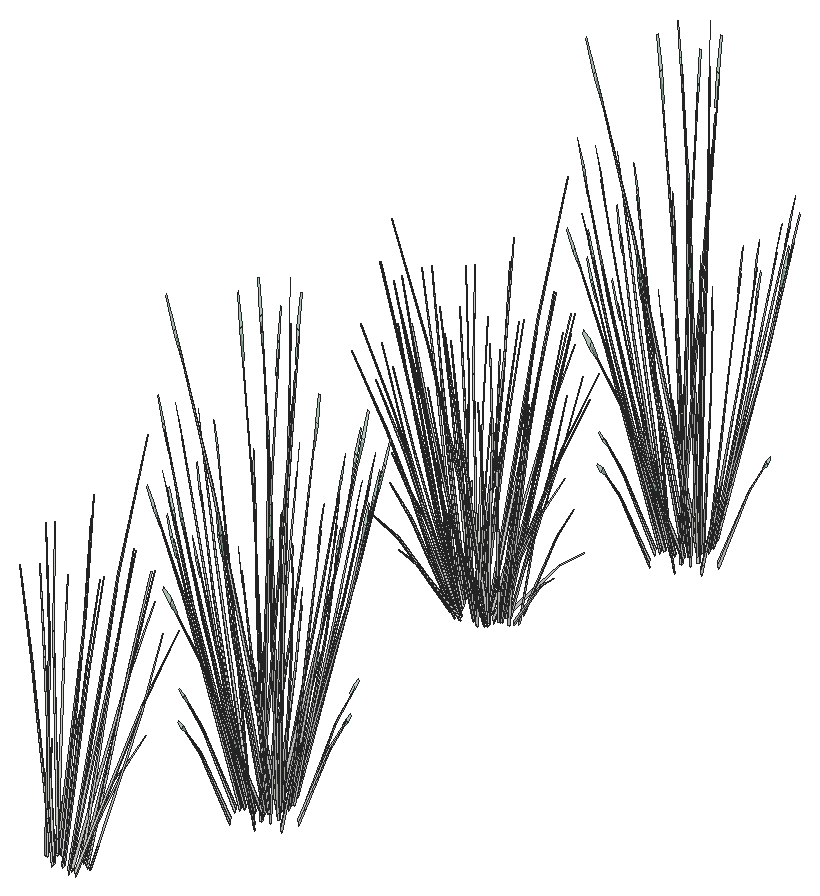
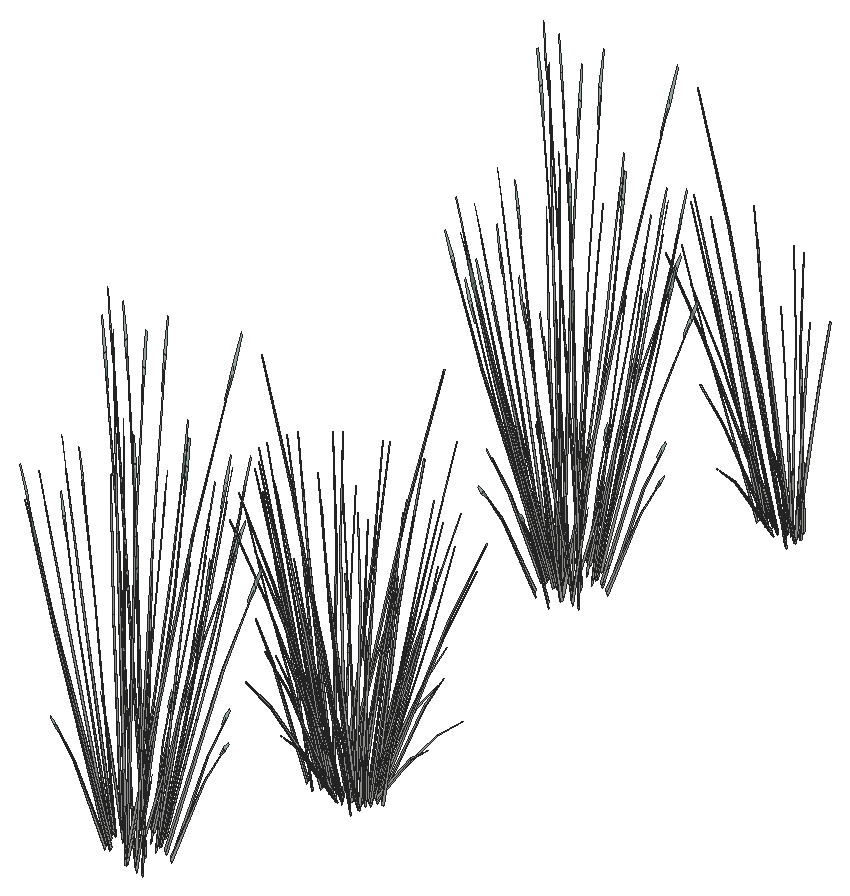
# SketchUp Ruby script. Lengths in inches.
U = 1.inch
M = Sketchup.active_model
def pt(a) = Geom::Point3d.new(a.map { |v| v * U })
def face(e, loops, mat)
  f = e.add_face(loops[0].map { |a| pt(a) })
  loops[1..].each { |l| e.add_face(l.map { |a| pt(a) }).erase! }
  f.material = f.back_material = mat if mat
  f
end
# faces: each face lists its corners as indices into pts; further lists are holes
def faces(e, pts, list, mat = nil) = list.each { |f| face(e, (f[0].is_a?(Array) ? f : [f]).map { |l| l.map { |i| pts[i] } }, mat) }
# xy, xz, yz: faces in a plane at the given z, y or x. An outline is a flat list of corners, or four numbers for a rectangle; further outlines are holes
def ring(l) = l.size == 4 ? [[l[0], l[1]], [l[2], l[1]], [l[2], l[3]], [l[0], l[3]]] : l.each_slice(2).to_a
def flat(e, list, mat, &to3) = list.each { |f| face(e, (f[0].is_a?(Array) ? f : [f]).map { |l| ring(l).map { |u, v| to3.(u, v) } }, mat) }
def xy(e, z, list, mat = nil) = flat(e, list, mat) { |x, y| [x, y, z] }
def xz(e, y, list, mat = nil) = flat(e, list, mat) { |x, z| [x, y, z] }
def yz(e, x, list, mat = nil) = flat(e, list, mat) { |y, z| [x, y, z] }
def lines(e, pts, list) = list.each { |a, b| e.add_line(pt(pts[a]), pt(pts[b])) }
# prism: a flat outline (further loops are holes) pulled along v
def prism(e, loops, v, mat = nil)
  f = face(e, loops, mat); d = Geom::Vector3d.new(v.map { |x| x * U })
  f.pushpull(f.normal.samedirection?(d) ? d.length : -d.length)
end
def box(e, o, s, mat = nil) = prism(e, [[o, [o[0] + s[0], o[1], o[2]], [o[0] + s[0], o[1] + s[1], o[2]], [o[0], o[1] + s[1], o[2]]]], [0, 0, s[2]], mat)
def at(x, y, z, deg = 0) = Geom::Transformation.translation(pt([x, y, z])) * Geom::Transformation.rotation(ORIGIN, Z_AXIS, deg.degrees)
def axes(o, x, y, z) = Geom::Transformation.new([*x, 0, *y, 0, *z, 0, *pt(o).to_a, 1])
def part(name) = M.definitions.add(name)
# library, detail: a bought-in or finely detailed component or shape, given as its bounding box
def library(name, o, s) = part(name).tap { |d| box(d.entities, o, s) }
def detail(e, o, s) = box(e.add_group.entities, o, s)
def put(e, d, t, mat = nil) = e.add_instance(d, t).tap { |i| i.material = mat if mat }
def group(e, t, mat = nil) = e.add_group.tap { |g| g.transformation = t; g.material = mat if mat }.entities
root = M.entities
M.materials.add("LightPink_Translucent").color = [175, 214, 192]
M.materials["LightPink_Translucent"].alpha = 0.75
c1 = part("blade")
p = [[2.15,0.21,22],[0,0.17,0],[0.09,0.45,0],[2.18,0.31,22],[2.29,0.31,22],[0.38,0.45,0],
  [2.48,0.24,33],[2.49,0.24,33],[2.48,0.22,33]]
faces(c1.entities,p,[[0,1,2,3],[4,5,2,3],[6,3,4,7],[8,0,3,6]])
c2 = part("blade with seeds\#1")
put(c2.entities,c1,at(0,0,0))
c3 = part("seeds")
p = [[0.3,-0.1,1.38],[-0.01,-0.03,1.59],[-0.01,-0.03,0.03],[0.14,-0.07,-0.07],[0.29,-0.03,3],[0.15,0.01,3.11]]
faces(c3.entities,p,[[0,1,2,3],[1,0,4,5]],"LightPink_Translucent")
c4 = part("blade with seeds")
put(c4.entities,c1,at(0,0,0))
put(c4.entities,c3,axes([2.4,0.25,30.99],[1.5799,-0.05474,1.17369],[-0.12525,1.92788,0.29478],[-0.07173,-0.02425,1.56792]))
put(root,c2,axes([488.05,398.95,140.43],[0.28286,0.23857,-0.29052],[-0.32298,0.22584,0.37506],[0.1641,0.03436,0.71765]))
put(root,c2,axes([487.94,398.95,140.6],[-0.36656,0.25108,0.39379],[-0.31614,-0.26664,0.3247],[0.17198,0.04631,0.81485]))
put(root,c2,axes([487.07,397.47,140.39],[-0.42958,-0.19798,1.1344],[0.45359,-0.30825,0.48946],[0.1386,0.18577,1.09651]))
put(root,c2,axes([487.04,398.34,139.9],[-0.18466,-0.06565,1.40588],[0.38215,-0.27542,0.11368],[0.23818,0.12424,0.601]))
put(root,c2,axes([483.98,398.31,140.85],[0.45986,0.21011,-0.09976],[-0.26493,0.30427,-0.55369],[-0.12992,0.10577,0.84132]))
put(root,c2,axes([484.6,398.21,139.9],[0.12417,-0.11708,1.40588],[0.31352,0.31602,0.11368],[-0.21504,0.14392,0.601]))
put(root,c2,axes([486.74,399.4,140.85],[0.29624,-0.32616,-0.09976],[0.42901,0.1879,-0.55369],[0.14913,0.09215,0.84132]))
put(root,c2,axes([486.35,399.67,140.58],[0.00147,-0.04613,1.45516],[0.42603,-0.20353,-0.1375],[0.14798,0.07265,0.25751]))
put(root,c2,axes([484.61,399.16,140.6],[-0.354,-0.25999,0.39379],[0.37594,-0.22422,0.3247],[-0.0653,0.12198,0.81485]))
put(root,c2,axes([486.94,399.45,140.6],[-0.49445,0.08745,0.39379],[-0.08581,-0.34303,0.3247],[0.11629,0.1011,0.81485]))
put(root,c2,axes([484.5,398.5,139.9],[0.09256,-0.13097,1.40588],[0.38832,0.27104,0.11368],[-0.17518,0.16893,0.601]))
put(root,c2,axes([484.61,399.24,140.43],[-0.33637,0.20062,-0.29052],[-0.31842,-0.22908,0.37506],[-0.04845,0.11639,0.71765]))
put(root,c2,axes([483.45,399.18,140.59],[-0.01236,0.0754,1.43516],[0.35069,0.26232,-0.22697],[-0.09181,0.12405,0.1151]))
put(root,c2,axes([484.57,399.01,141.15],[0.54637,0.01888,-0.11073],[-0.01493,0.35746,-0.6146],[-0.03795,0.13767,0.93387]))
put(root,c2,axes([485.58,399.41,140.85],[0.48648,-0.17741,-0.09976],[0.23906,0.31487,-0.55369],[0.06419,0.13269,0.84132]))
put(root,c2,axes([484.94,399.15,140.82],[0.35588,0.25603,-0.4653],[-0.37594,0.22422,-0.36041],[-0.05415,0.13008,0.89031]))
put(root,c2,axes([486.28,398.72,139.9],[-0.11364,-0.12234,1.40588],[0.52511,-0.103,0.11368],[0.11868,0.19206,0.601]))
put(root,c2,axes([485.78,399.59,140.43],[-0.14987,0.29303,-0.29052],[-0.43725,-0.08547,0.37506],[0.04009,0.11798,0.71765]))
put(root,c2,axes([485.35,398.78,139.9],[-0.01217,-0.14625,1.40588],[0.52737,0.09702,0.11368],[-0.03262,0.20842,0.601]))
put(root,c2,axes([483.41,399.95,140.58],[0.0564,-0.02301,1.45516],[0.46615,0.15302,-0.1375],[-0.01095,0.12741,0.25751]))
put(root,c2,axes([485.47,400.11,140.59],[0.06302,0.06136,1.43516],[0.50855,0.02411,-0.22697],[0.05114,0.13532,0.1151]))
put(root,c2,axes([484.65,399.52,139.48],[0.01092,-0.19671,1.26617],[0.49126,0.1039,0.17497],[-0.04257,0.20964,0.59789]))
put(root,c4,axes([493.37,414.48,140.21],[0.06442,0.13585,1.61128],[-0.4498,0.04685,0.1261],[-0.05969,-0.29426,0.57588]))
put(root,c4,axes([494.09,414.04,141.7],[0.01072,-0.47777,-0.64651],[0.45152,0.03209,0.07802],[0.04765,-0.2024,0.91455]))
put(root,c4,axes([493.3125,413.27,141.29],[0.12423,-0.3972,-0.32227],[0.36244,0.11585,0.41605],[-0.03323,-0.15992,0.79608]))
put(root,c4,axes([493.125,413.55,141.43],[-0.40508,-0.12948,-0.465],[0.13885,-0.44393,-0.36018],[-0.03714,-0.17873,0.88973]))
put(root,c4,axes([494,413.88,141.43],[-0.29499,-0.34704,-0.465],[0.31162,-0.30393,-0.36018],[0.04488,-0.17633,0.88973]))
put(root,c4,axes([491.39,412.67,139.6875],[0.20183,0.19918,1.04523],[-0.31952,0.0786,0.76796],[-0.05721,-0.14394,0.23022]))
put(root,c4,axes([494.28,413.75,141.29],[0.27882,-0.27194,-0.32227],[0.26394,0.31051,0.41605],[0.04016,-0.15777,0.79608]))
put(root,c4,axes([492.27,413.42,141.29],[-0.06364,-0.41603,-0.32227],[0.36383,-0.10985,0.41605],[-0.09772,-0.11922,0.79608]))
put(root,c4,axes([493.61,413.1,139.6875],[0.03187,0.30513,1.04523],[-0.28077,-0.19355,0.76796],[0.04212,-0.15079,0.23022]))
put(root,c4,axes([492.22,413.76,141.43],[-0.40663,0.12278,-0.465],[-0.07113,-0.46497,-0.36018],[-0.10922,-0.13325,0.88973]))
put(root,c4,axes([494.625,414.87,141.7],[0.21525,-0.40754,-0.64651],[0.37719,0.28963,0.07802],[0.12852,-0.14765,0.91455]))
put(root,c4,axes([494.61,414.68,141.43],[-0.10586,-0.47162,-0.465],[0.4009,-0.0825,-0.36018],[0.11489,-0.12667,0.88973]))
put(root,c4,axes([494.91,414.73,141.29],[0.3587,-0.07382,-0.32227],[0.09472,0.42197,0.41605],[0.10279,-0.11334,0.79608]))
put(root,c4,axes([491.42,414.15,141.29],[-0.23447,-0.32338,-0.32227],[0.26773,-0.30612,0.41605],[-0.13603,-0.04658,0.79608]))
put(root,c4,axes([492.19,415.85,140.2],[-0.17958,0.41302,1.37647],[-0.38687,-0.40462,0.54432],[0.22929,-0.18124,1.15394]))
put(root,c4,axes([495.45,414.27,139.6875],[-0.155,0.24931,1.04523],[-0.09317,-0.36309,0.76796],[0.11912,-0.07769,0.23022]))
put(root,c4,axes([491.67,414.37,142.03],[-0.41193,-0.01244,-0.71763],[0.02767,-0.52368,0.0866],[-0.17451,-0.05527,1.01516]))
put(root,c4,axes([490.51,414.36,139.6875],[0.2648,-0.01237,1.04523],[-0.18886,0.30908,0.76796],[-0.12621,-0.06079,0.23022]))
put(root,c4,axes([491.09,414.19,140.23],[0.22989,0.0105,1.40454],[-0.12143,0.4723,0.19409],[-0.24501,-0.04092,0.66323]))
put(root,c4,axes([491.54,414.47,141.72],[-0.29922,0.34214,-0.51615],[-0.26205,-0.36143,-0.3998],[-0.15203,-0.05206,0.9876]))
put(root,c4,axes([493.05,416.49,139.76],[0.4193,-0.01306,1.28558],[-0.10869,0.59089,0.54432],[-0.22943,-0.13975,1.21348]))
put(root,c4,axes([494.8,415.73,141.43],[0.11164,-0.46982,-0.465],[0.38276,0.16104,-0.36018],[0.1541,-0.04308,0.88973]))
put(root,c4,axes([492.79,415.13,139.64],[-0.40128,-0.23189,0.40713],[0.19312,-0.48183,-0.19594],[0.0925,0,1.30716]))
put(root,c4,axes([494.73,415.9,141.7],[0.3621,-0.22811,-0.64651],[0.2018,0.46957,0.07802],[0.17496,-0.05334,0.91455]))
put(root,c4,axes([492.61,416.25,139.64],[0.02749,0.519,0.40713],[-0.45634,0.04694,-0.19594],[-0.04625,-0.09291,1.30716]))
put(root,c4,axes([495.04,415.94,141.29],[0.34247,0.14409,-0.32227],[-0.09989,0.42037,0.41605],[0.13788,-0.03855,0.79608]))
put(root,c4,axes([491.01,415.27,141.29],[-0.34247,-0.14409,-0.32227],[0.09989,-0.42037,0.41605],[-0.13788,0.03855,0.79608]))
put(root,c4,axes([493.35,415.26,139.64],[-0.02749,-0.519,0.40713],[0.45634,-0.04694,-0.19594],[0.04625,0.09291,1.30716]))
put(root,c4,axes([491.32,415.32,141.7],[-0.3621,0.22811,-0.64651],[-0.2018,-0.46957,0.07802],[-0.17496,0.05334,0.91455]))
put(root,c4,axes([495.76,416.02,139.6875],[-0.25968,0.06131,1.04523],[0.14383,-0.34012,0.76796],[0.13297,0.0366,0.23022]))
put(root,c4,axes([493.17,416.375,139.64],[0.40128,0.23189,0.40713],[-0.19312,0.48183,-0.19594],[-0.0925,0,1.30716]))
put(root,c4,axes([491.25,415.49,141.43],[-0.11164,0.46982,-0.465],[-0.38276,-0.16104,-0.36018],[-0.1541,0.04308,0.88973]))
put(root,c4,axes([493.54,415.88,139.64],[0.37379,-0.28711,0.40713],[0.26322,0.43489,-0.19594],[-0.04625,0.09291,1.30716]))
put(root,c4,axes([494.51,416.74,141.43],[0.29922,-0.34214,-0.465],[0.26205,0.36143,-0.36018],[0.15203,0.05206,0.88973]))
put(root,c4,axes([494.375,416.85,141.7],[0.41193,0.01244,-0.64651],[-0.02767,0.52368,0.07802],[0.17451,0.05527,0.91455]))
put(root,c4,axes([494.62,417.07,141.29],[0.23447,0.32338,-0.32227],[-0.26773,0.30612,0.41605],[0.13603,0.04658,0.79608]))
put(root,c4,axes([491.61,417.14,139.6875],[0.12805,-0.2691,1.04523],[0.13011,0.34747,0.76796],[-0.11021,0.09372,0.23022]))
put(root,c4,axes([491.02,417.1875,139.6],[0.01397,-0.30649,0.95605],[0.29664,0.2024,0.52785],[-0.10539,0.12108,0.74993]))
put(root,c4,axes([491.43,416.53,141.43],[0.10586,0.47162,-0.465],[-0.4009,0.0825,-0.36018],[-0.11489,0.12667,0.88973]))
put(root,c4,axes([493.82,417.45,141.43],[0.40663,-0.12278,-0.465],[0.07113,0.46497,-0.36018],[0.10922,0.13325,0.88973]))
put(root,c4,axes([491.72,418.27,140.75],[0.37435,-0.09148,-0.03177],[0.08606,0.43236,-0.14407],[-0.02373,0.09029,0.47519]))
put(root,c4,axes([494.63,418.02,139.6875],[-0.2267,-0.15919,1.04523],[0.30457,-0.13683,0.76796],[0.07632,0.13148,0.23022]))
put(root,c4,axes([493.78,417.8,141.29],[0.06364,0.41603,-0.32227],[-0.36383,0.10985,0.41605],[0.09772,0.11922,0.79608]))
put(root,c4,axes([493.66,417.47,141.7],[0.35138,0.24965,-0.64651],[-0.24972,0.43748,0.07802],[0.12731,0.14906,0.91455]))
put(root,c4,axes([491.77,417.46,141.29],[-0.27882,0.27194,-0.32227],[-0.26394,-0.31051,0.41605],[-0.04016,0.15777,0.79608]))
put(root,c4,axes([492.92,417.67,141.43],[0.40508,0.12948,-0.465],[-0.13885,0.44393,-0.36018],[0.03714,0.17873,0.88973]))
put(root,c4,axes([492.66,418.78,139.6875],[-0.07352,-0.2953,1.04523],[0.30384,0.139,0.76796],[-0.02079,0.15666,0.23022]))
put(root,c4,axes([492.73,417.94,141.29],[-0.12423,0.3972,-0.32227],[-0.36244,-0.11585,0.41605],[0.03323,0.15992,0.79608]))
put(root,c4,axes([491.95,417.17,141.7],[-0.01072,0.47777,-0.64651],[-0.45152,-0.03209,0.07802],[-0.04765,0.2024,0.91455]))
put(root,c4,axes([492.77,417.59,141.7],[0.19668,0.41997,-0.64651],[-0.40486,0.23405,0.07802],[0.04599,0.20292,0.91455]))
put(root,c2,axes([485.03,449.9,139.9],[0.11364,0.12234,1.40588],[-0.52511,0.103,0.11368],[-0.11868,-0.19206,0.601]))
put(root,c2,axes([485.9,449.08,140.59],[-0.07604,-0.05342,1.43516],[-0.50744,0.03387,-0.22697],[-0.08099,-0.12778,0.1151]))
put(root,c2,axes([488.07,449.47,140.58],[-0.05049,0.0291,1.45516],[-0.49465,-0.09819,-0.1375],[-0.01791,-0.12701,0.25751]))
put(root,c2,axes([488.18,449.74,140.59],[-0.0048,-0.07584,1.43516],[-0.40531,-0.21918,-0.22697],[0.06266,-0.13286,0.1151]))
put(root,c2,axes([486.8,450.11,139.9],[-0.09256,0.13097,1.40588],[-0.38832,-0.27104,0.11368],[0.17518,-0.16893,0.601]))
put(root,c2,axes([486.47,449.72,140.43],[0.14987,-0.29303,-0.29052],[0.43725,0.08547,0.37506],[-0.04009,-0.11798,0.71765]))
put(root,c2,axes([485.375,448.91,140.58],[-0.00927,0.04567,1.45516],[-0.45742,0.16576,-0.1375],[-0.1346,-0.08473,0.25751]))
put(root,c2,axes([486.67,449.91,140.85],[-0.48648,0.17741,-0.09976],[-0.23906,-0.31487,-0.55369],[-0.06419,-0.13269,0.84132]))
put(root,c2,axes([486.53,449.79,140.6],[0.48986,0.09962,0.39379],[-0.16751,0.3275,0.3247],[-0.02944,-0.12879,0.81485]))
put(root,c2,axes([487.68,450.31,140.85],[-0.54637,-0.01888,-0.09976],[0.01493,-0.35746,-0.55369],[0.03795,-0.13767,0.84132]))
put(root,c2,axes([485.21,449.83,140.43],[-0.07678,-0.30692,-0.29052],[0.43892,-0.08104,0.37506],[-0.11789,-0.08795,0.71765]))
put(root,c2,axes([487.64,450.08,140.43],[0.33637,-0.20062,-0.29052],[0.31842,0.22908,0.37506],[0.04845,-0.11639,0.71765]))
put(root,c2,axes([484.27,450.28,139.9],[0.18466,0.06565,1.40588],[-0.38215,0.27542,0.11368],[-0.23818,-0.12424,0.601]))
put(root,c2,axes([485.5,449.78,141.17],[-0.33178,0.3653,-0.11173],[-0.48049,-0.21045,-0.62013],[-0.16702,-0.10321,0.94228]))
put(root,c2,axes([487.64,450.16,140.6],[0.354,0.25999,0.39379],[-0.37594,0.22422,0.3247],[0.0653,-0.12198,0.81485]))
put(root,c2,axes([484.23,449.67,140.59],[-0.10696,-0.00269,1.43516],[-0.34054,0.26896,-0.22697],[-0.1817,-0.05496,0.1151]))
put(root,c2,axes([488.27,451.01,140.85],[-0.45986,-0.21011,-0.09976],[0.26493,-0.30427,-0.55369],[0.12992,-0.10577,0.84132]))
put(root,c2,axes([489.41,450.92,140.58],[-0.06493,-0.00289,1.45516],[-0.26964,-0.31009,-0.1375],[0.10828,-0.10196,0.25751]))
put(root,c2,axes([486.375,452.16,139.45],[0.4296,0.15365,1.24087],[-0.42086,0.33102,0.4907],[-0.18851,-0.19619,1.04025]))
put(root,c2,axes([484.2,450.37,140.43],[-0.28286,-0.23857,-0.29052],[0.32298,-0.22584,0.37506],[-0.1641,-0.03436,0.71765]))
put(root,c2,axes([488.4,450.8,140.43],[0.43273,-0.05446,-0.29052],[0.11427,0.31131,0.37506],[0.12401,-0.08362,0.71765]))
put(root,c2,axes([488.35,450.87,140.6],[0.12329,0.35069,0.39379],[-0.48364,0.06086,0.3247],[0.14254,-0.08248,0.81485]))
put(root,c2,axes([489.65,451.29,140.59],[0.06898,-0.05804,1.43516],[-0.0883,-0.35603,-0.22697],[0.17309,-0.0675,0.1151]))
put(root,c2,axes([483.82,449.9,140.58],[0.03685,0.03803,1.45516],[-0.17767,0.34183,-0.1375],[-0.17994,0.00247,0.25751]))
put(root,c2,axes([484.52,450.34,140.85],[-0.02662,0.38751,-0.09976],[-0.50399,-0.01059,-0.55369],[-0.19411,-0.02692,0.84132]))
put(root,c2,axes([488.29,451.83,140.85],[-0.25013,-0.34504,-0.09976],[0.44394,-0.16956,-0.55369],[0.18708,-0.04552,0.84132]))
put(root,c2,axes([483.88,450.88,139.9],[0.2062,-0.00863,1.40588],[-0.13679,0.37404,0.11368],[-0.29386,-0.02314,0.601]))
put(root,c2,axes([483.79,451.16,140.6],[0.14045,-0.34743,0.39379],[0.46175,0.1188,0.3247],[-0.18159,0.02088,0.81485]))
put(root,c2,axes([483.7,451.2,140.43],[-0.41315,-0.1063,-0.29052],[0.1205,-0.31012,0.37506],[-0.16634,0.02844,0.71765]))
put(root,c2,axes([488.55,451.69,140.43],[0.41315,0.1063,-0.29052],[-0.1205,0.31012,0.37506],[0.16634,-0.02844,0.71765]))
put(root,c2,axes([487.43,451.31,139.9],[-0.2062,0.00863,1.40588],[0.13679,-0.37404,0.11368],[0.29386,0.02314,0.601]))
put(root,c2,axes([488.46,451.73,140.6],[-0.14045,0.34743,0.39379],[-0.46175,-0.1188,0.3247],[0.18159,-0.02088,0.81485]))
put(root,c2,axes([483.96,451.0625,140.85],[0.25013,0.34504,-0.09976],[-0.44394,0.16956,-0.55369],[-0.18708,0.04552,0.84132]))
put(root,c2,axes([489.29,452.86,140.58],[-0.04495,-0.03336,1.45516],[0.09833,-0.35758,-0.1375],[0.17707,-0.02285,0.25751]))
put(root,c2,axes([483.4375,451.41,140.59],[-0.08118,0.04947,1.43516],[0.00691,0.36146,-0.22697],[-0.18608,0.04701,0.1151]))
put(root,c2,axes([488.9,452.56,139.94],[-0.09515,-0.32031,-0.02864],[0.44972,-0.07364,-0.12987],[0.09391,0.02031,0.42837]))
put(root,c2,axes([487.73,452.55,140.85],[0.02662,-0.38751,-0.09976],[0.50399,0.01059,-0.55369],[0.19411,0.02692,0.84132]))
put(root,c2,axes([488.17,452.32,140.59],[0.10664,-0.00644,1.43516],[0.29251,-0.29603,-0.22697],[0.18969,0.03908,0.1151]))
put(root,c2,axes([483.9,452.03,140.6],[-0.12329,-0.35069,0.39379],[0.48364,-0.06086,0.3247],[-0.14254,0.08248,0.81485]))
put(root,c2,axes([483.96,451.54,139.9],[0.17249,-0.0806,1.40588],[0.14522,0.37244,0.11368],[-0.2708,0.08417,0.601]))
put(root,c2,axes([482.53,451.77,140.58],[0.06344,0.01022,1.45516],[0.19627,0.33667,-0.1375],[-0.12987,0.08837,0.25751]))
put(root,c2,axes([483.85,452.09,140.43],[-0.43273,0.05446,-0.29052],[-0.11427,-0.31131,0.37506],[-0.12401,0.08362,0.71765]))
put(root,c2,axes([488.05,452.52,140.43],[0.28286,0.23857,-0.29052],[-0.32298,0.22584,0.37506],[0.1641,0.03436,0.71765]))
put(root,c2,axes([487.94,452.52,140.6],[-0.36656,0.25108,0.39379],[-0.31614,-0.26664,0.3247],[0.17198,0.04631,0.81485]))
put(root,c2,axes([487.07,451.05,140.39],[-0.42958,-0.19798,1.1344],[0.45359,-0.30825,0.48946],[0.1386,0.18577,1.09651]))
put(root,c2,axes([487.04,451.91,139.9],[-0.18466,-0.06565,1.40588],[0.38215,-0.27542,0.11368],[0.23818,0.12424,0.601]))
put(root,c2,axes([483.98,451.88,140.85],[0.45986,0.21011,-0.09976],[-0.26493,0.30427,-0.55369],[-0.12992,0.10577,0.84132]))
put(root,c2,axes([484.6,451.79,139.9],[0.12417,-0.11708,1.40588],[0.31352,0.31602,0.11368],[-0.21504,0.14392,0.601]))
put(root,c2,axes([486.74,452.97,140.85],[0.29624,-0.32616,-0.09976],[0.42901,0.1879,-0.55369],[0.14913,0.09215,0.84132]))
put(root,c2,axes([486.35,453.24,140.58],[0.00147,-0.04613,1.45516],[0.42603,-0.20353,-0.1375],[0.14798,0.07265,0.25751]))
put(root,c2,axes([484.61,452.74,140.6],[-0.354,-0.25999,0.39379],[0.37594,-0.22422,0.3247],[-0.0653,0.12198,0.81485]))
put(root,c2,axes([486.94,453.02,140.6],[-0.49445,0.08745,0.39379],[-0.08581,-0.34303,0.3247],[0.11629,0.1011,0.81485]))
put(root,c2,axes([484.5,452.08,139.9],[0.09256,-0.13097,1.40588],[0.38832,0.27104,0.11368],[-0.17518,0.16893,0.601]))
put(root,c2,axes([484.61,452.8125,140.43],[-0.33637,0.20062,-0.29052],[-0.31842,-0.22908,0.37506],[-0.04845,0.11639,0.71765]))
put(root,c2,axes([483.45,452.75,140.59],[-0.01236,0.0754,1.43516],[0.35069,0.26232,-0.22697],[-0.09181,0.12405,0.1151]))
put(root,c2,axes([484.57,452.58,141.15],[0.54637,0.01888,-0.11073],[-0.01493,0.35746,-0.6146],[-0.03795,0.13767,0.93387]))
put(root,c2,axes([485.58,452.98,140.85],[0.48648,-0.17741,-0.09976],[0.23906,0.31487,-0.55369],[0.06419,0.13269,0.84132]))
put(root,c2,axes([484.94,452.72,140.82],[0.35588,0.25603,-0.4653],[-0.37594,0.22422,-0.36041],[-0.05415,0.13008,0.89031]))
put(root,c2,axes([486.28,452.29,139.9],[-0.11364,-0.12234,1.40588],[0.52511,-0.103,0.11368],[0.11868,0.19206,0.601]))
put(root,c2,axes([485.78,453.17,140.43],[-0.14987,0.29303,-0.29052],[-0.43725,-0.08547,0.37506],[0.04009,0.11798,0.71765]))
put(root,c2,axes([485.35,452.35,139.9],[-0.01217,-0.14625,1.40588],[0.52737,0.09702,0.11368],[-0.03262,0.20842,0.601]))
put(root,c2,axes([483.41,453.53,140.58],[0.0564,-0.02301,1.45516],[0.46615,0.15302,-0.1375],[-0.01095,0.12741,0.25751]))
put(root,c2,axes([485.47,453.6875,140.59],[0.06302,0.06136,1.43516],[0.50855,0.02411,-0.22697],[0.05114,0.13532,0.1151]))
put(root,c2,axes([484.65,453.1,139.48],[0.01092,-0.19671,1.26617],[0.49126,0.1039,0.17497],[-0.04257,0.20964,0.59789]))
put(root,c4,axes([493.37,468.06,140.21],[0.06442,0.13585,1.61128],[-0.4498,0.04685,0.1261],[-0.05969,-0.29426,0.57588]))
put(root,c4,axes([494.09,467.61,141.7],[0.01072,-0.47777,-0.64651],[0.45152,0.03209,0.07802],[0.04765,-0.2024,0.91455]))
put(root,c4,axes([493.3125,466.85,141.29],[0.12423,-0.3972,-0.32227],[0.36244,0.11585,0.41605],[-0.03323,-0.15992,0.79608]))
put(root,c4,axes([493.125,467.12,141.43],[-0.40508,-0.12948,-0.465],[0.13885,-0.44393,-0.36018],[-0.03714,-0.17873,0.88973]))
put(root,c4,axes([494,467.46,141.43],[-0.29499,-0.34704,-0.465],[0.31162,-0.30393,-0.36018],[0.04488,-0.17633,0.88973]))
put(root,c4,axes([491.39,466.24,139.6875],[0.20183,0.19918,1.04523],[-0.31952,0.0786,0.76796],[-0.05721,-0.14394,0.23022]))
put(root,c4,axes([494.28,467.33,141.29],[0.27882,-0.27194,-0.32227],[0.26394,0.31051,0.41605],[0.04016,-0.15777,0.79608]))
put(root,c4,axes([492.27,466.99,141.29],[-0.06364,-0.41603,-0.32227],[0.36383,-0.10985,0.41605],[-0.09772,-0.11922,0.79608]))
put(root,c4,axes([493.61,466.67,139.6875],[0.03187,0.30513,1.04523],[-0.28077,-0.19355,0.76796],[0.04212,-0.15079,0.23022]))
put(root,c4,axes([492.22,467.34,141.43],[-0.40663,0.12278,-0.465],[-0.07113,-0.46497,-0.36018],[-0.10922,-0.13325,0.88973]))
put(root,c4,axes([494.625,468.45,141.7],[0.21525,-0.40754,-0.64651],[0.37719,0.28963,0.07802],[0.12852,-0.14765,0.91455]))
put(root,c4,axes([494.61,468.25,141.43],[-0.10586,-0.47162,-0.465],[0.4009,-0.0825,-0.36018],[0.11489,-0.12667,0.88973]))
put(root,c4,axes([494.91,468.3,141.29],[0.3587,-0.07382,-0.32227],[0.09472,0.42197,0.41605],[0.10279,-0.11334,0.79608]))
put(root,c4,axes([491.42,467.72,141.29],[-0.23447,-0.32338,-0.32227],[0.26773,-0.30612,0.41605],[-0.13603,-0.04658,0.79608]))
put(root,c4,axes([492.19,469.42,140.2],[-0.17958,0.41302,1.37647],[-0.38687,-0.40462,0.54432],[0.22929,-0.18124,1.15394]))
put(root,c4,axes([495.45,467.84,139.6875],[-0.155,0.24931,1.04523],[-0.09317,-0.36309,0.76796],[0.11912,-0.07769,0.23022]))
put(root,c4,axes([491.67,467.94,142.03],[-0.41193,-0.01244,-0.71763],[0.02767,-0.52368,0.0866],[-0.17451,-0.05527,1.01516]))
put(root,c4,axes([490.51,467.93,139.6875],[0.2648,-0.01237,1.04523],[-0.18886,0.30908,0.76796],[-0.12621,-0.06079,0.23022]))
put(root,c4,axes([491.09,467.76,140.23],[0.22989,0.0105,1.40454],[-0.12143,0.4723,0.19409],[-0.24501,-0.04092,0.66323]))
put(root,c4,axes([491.54,468.05,141.72],[-0.29922,0.34214,-0.51615],[-0.26205,-0.36143,-0.3998],[-0.15203,-0.05206,0.9876]))
put(root,c4,axes([493.05,470.0625,139.76],[0.4193,-0.01306,1.28558],[-0.10869,0.59089,0.54432],[-0.22943,-0.13975,1.21348]))
put(root,c4,axes([494.8,469.3,141.43],[0.11164,-0.46982,-0.465],[0.38276,0.16104,-0.36018],[0.1541,-0.04308,0.88973]))
put(root,c4,axes([492.79,468.71,139.64],[-0.40128,-0.23189,0.40713],[0.19312,-0.48183,-0.19594],[0.0925,0,1.30716]))
put(root,c4,axes([494.73,469.47,141.7],[0.3621,-0.22811,-0.64651],[0.2018,0.46957,0.07802],[0.17496,-0.05334,0.91455]))
put(root,c4,axes([492.61,469.83,139.64],[0.02749,0.519,0.40713],[-0.45634,0.04694,-0.19594],[-0.04625,-0.09291,1.30716]))
put(root,c4,axes([495.04,469.52,141.29],[0.34247,0.14409,-0.32227],[-0.09989,0.42037,0.41605],[0.13788,-0.03855,0.79608]))
put(root,c4,axes([491.01,468.85,141.29],[-0.34247,-0.14409,-0.32227],[0.09989,-0.42037,0.41605],[-0.13788,0.03855,0.79608]))
put(root,c4,axes([493.35,468.83,139.64],[-0.02749,-0.519,0.40713],[0.45634,-0.04694,-0.19594],[0.04625,0.09291,1.30716]))
put(root,c4,axes([491.32,468.89,141.7],[-0.3621,0.22811,-0.64651],[-0.2018,-0.46957,0.07802],[-0.17496,0.05334,0.91455]))
put(root,c4,axes([495.76,469.59,139.6875],[-0.25968,0.06131,1.04523],[0.14383,-0.34012,0.76796],[0.13297,0.0366,0.23022]))
put(root,c4,axes([493.17,469.95,139.64],[0.40128,0.23189,0.40713],[-0.19312,0.48183,-0.19594],[-0.0925,0,1.30716]))
put(root,c4,axes([491.25,469.0625,141.43],[-0.11164,0.46982,-0.465],[-0.38276,-0.16104,-0.36018],[-0.1541,0.04308,0.88973]))
put(root,c4,axes([493.54,469.45,139.64],[0.37379,-0.28711,0.40713],[0.26322,0.43489,-0.19594],[-0.04625,0.09291,1.30716]))
put(root,c4,axes([494.51,470.32,141.43],[0.29922,-0.34214,-0.465],[0.26205,0.36143,-0.36018],[0.15203,0.05206,0.88973]))
put(root,c4,axes([494.375,470.42,141.7],[0.41193,0.01244,-0.64651],[-0.02767,0.52368,0.07802],[0.17451,0.05527,0.91455]))
put(root,c4,axes([494.62,470.64,141.29],[0.23447,0.32338,-0.32227],[-0.26773,0.30612,0.41605],[0.13603,0.04658,0.79608]))
put(root,c4,axes([491.61,470.72,139.6875],[0.12805,-0.2691,1.04523],[0.13011,0.34747,0.76796],[-0.11021,0.09372,0.23022]))
put(root,c4,axes([491.02,470.76,139.6],[0.01397,-0.30649,0.95605],[0.29664,0.2024,0.52785],[-0.10539,0.12108,0.74993]))
put(root,c4,axes([491.43,470.11,141.43],[0.10586,0.47162,-0.465],[-0.4009,0.0825,-0.36018],[-0.11489,0.12667,0.88973]))
put(root,c4,axes([493.82,471.03,141.43],[0.40663,-0.12278,-0.465],[0.07113,0.46497,-0.36018],[0.10922,0.13325,0.88973]))
